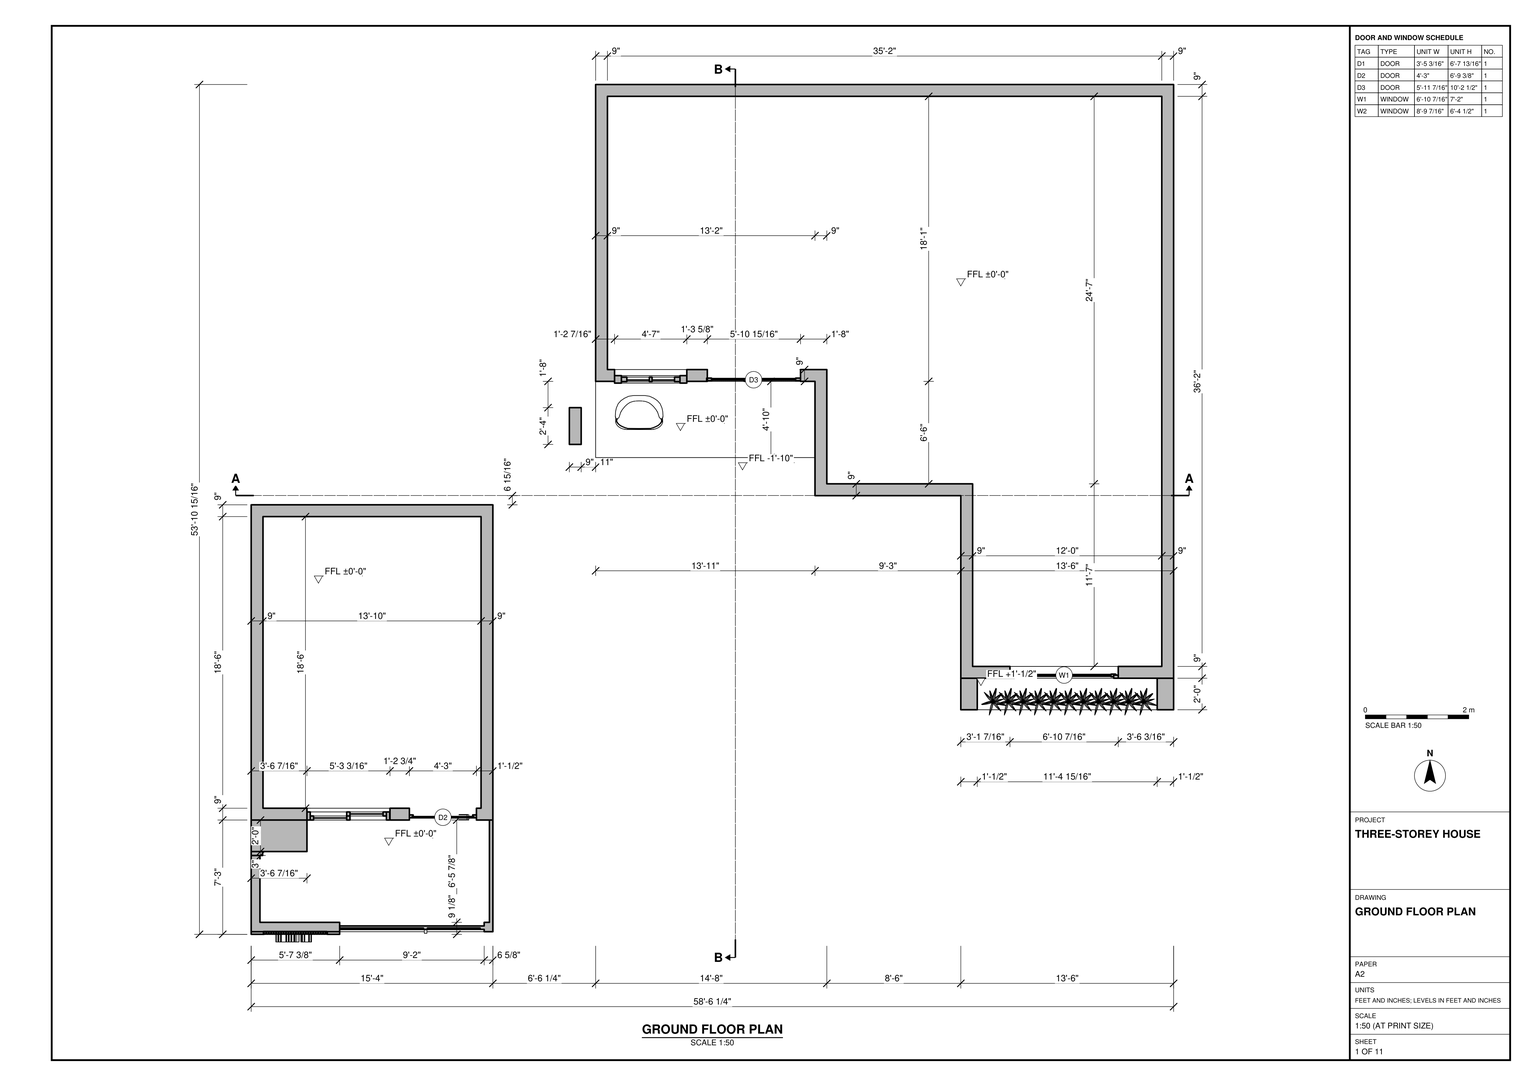
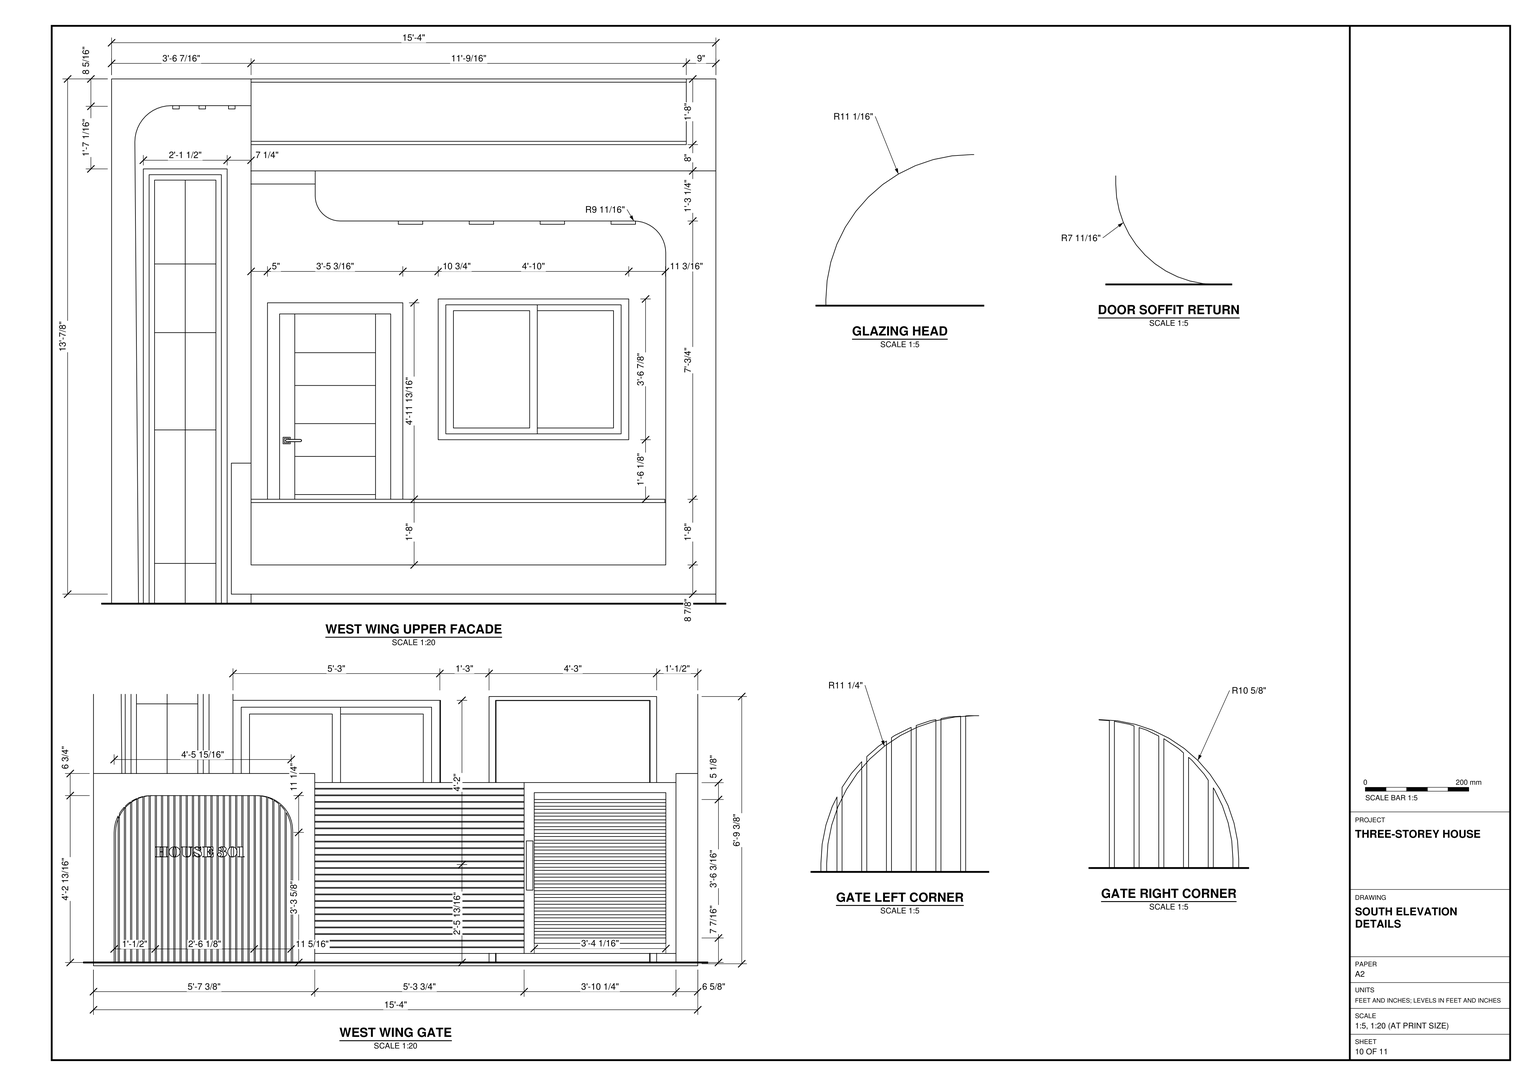
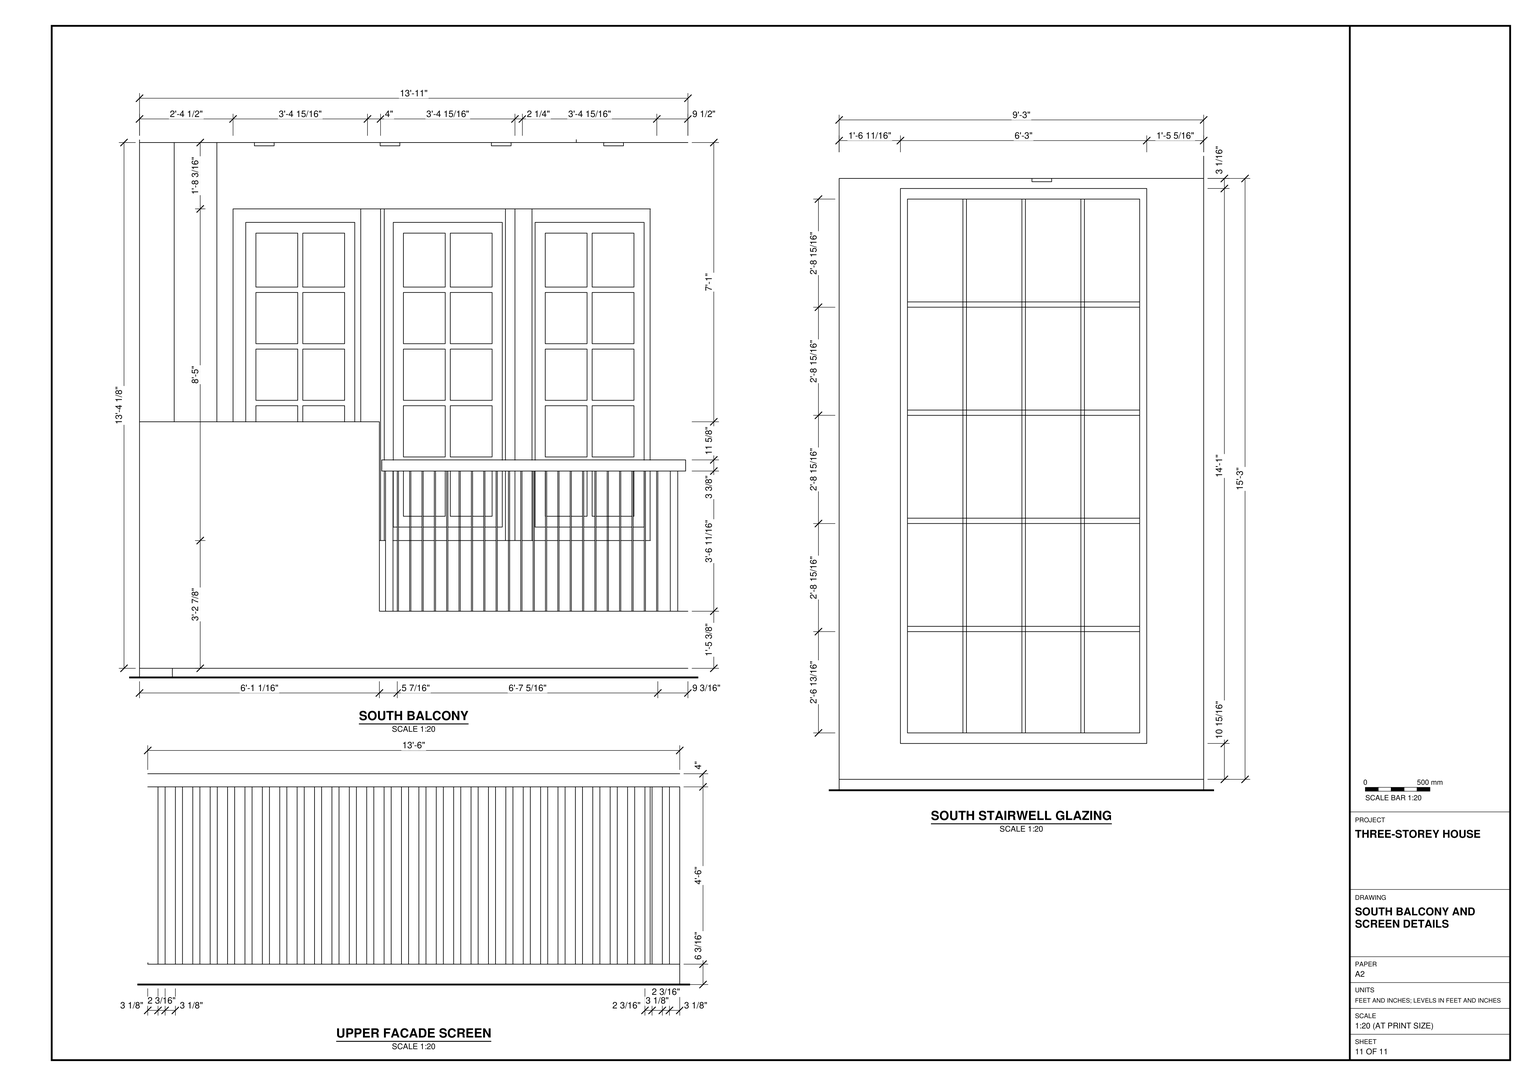
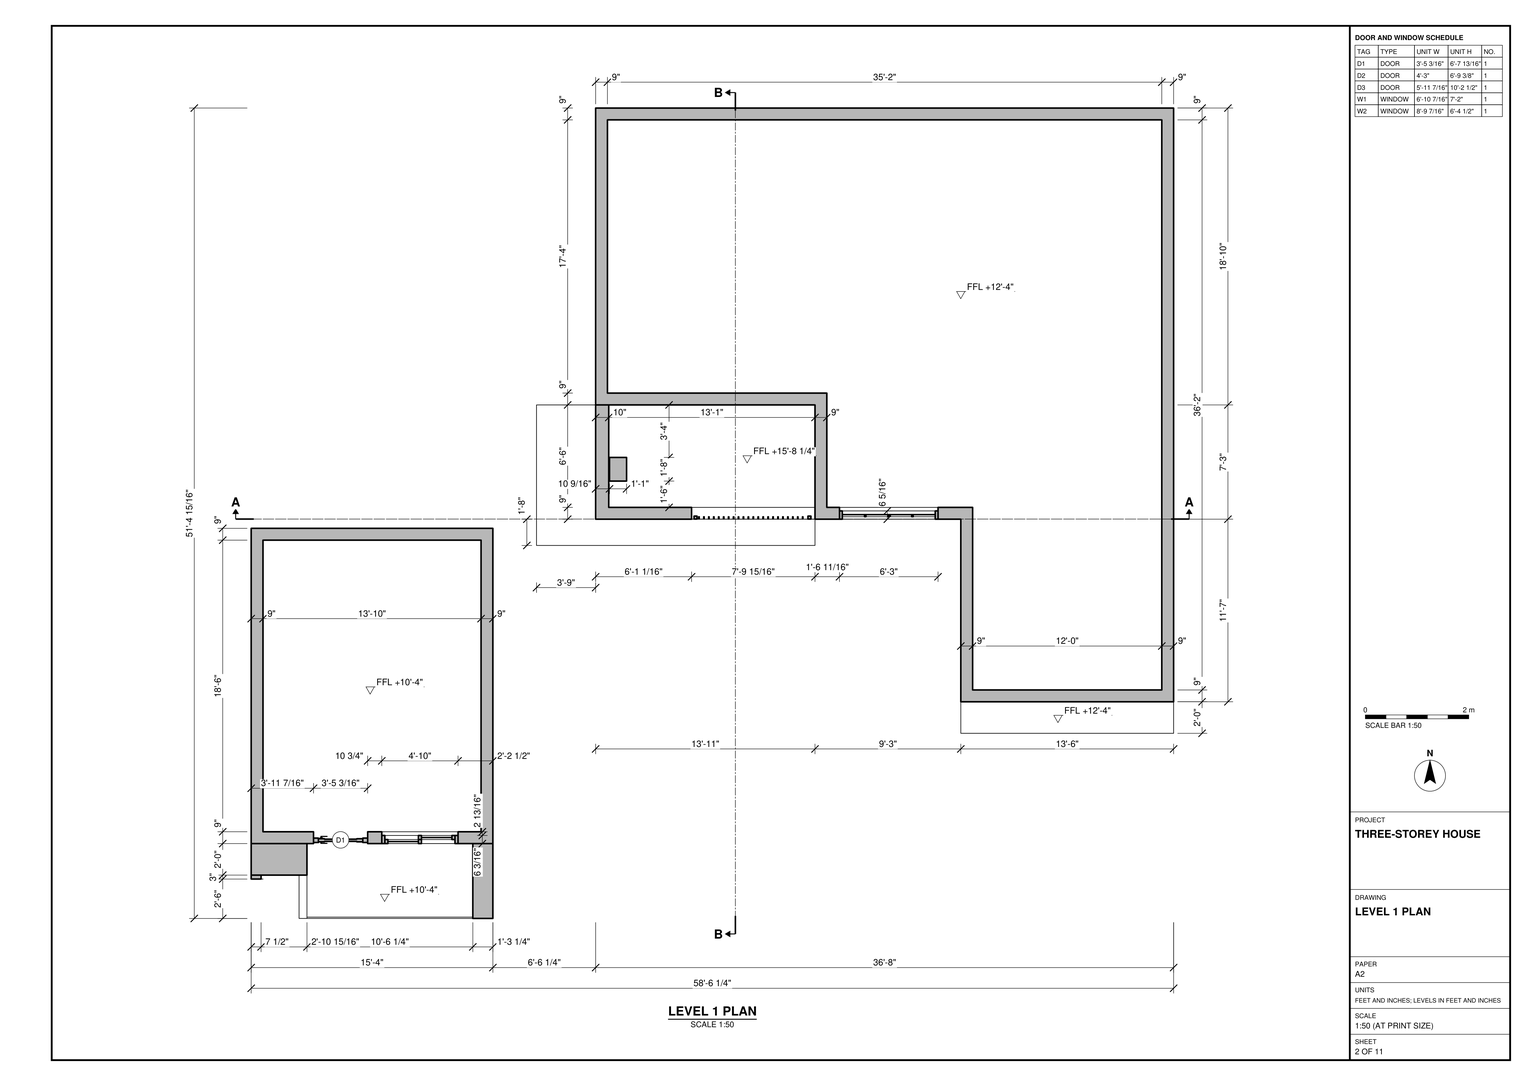
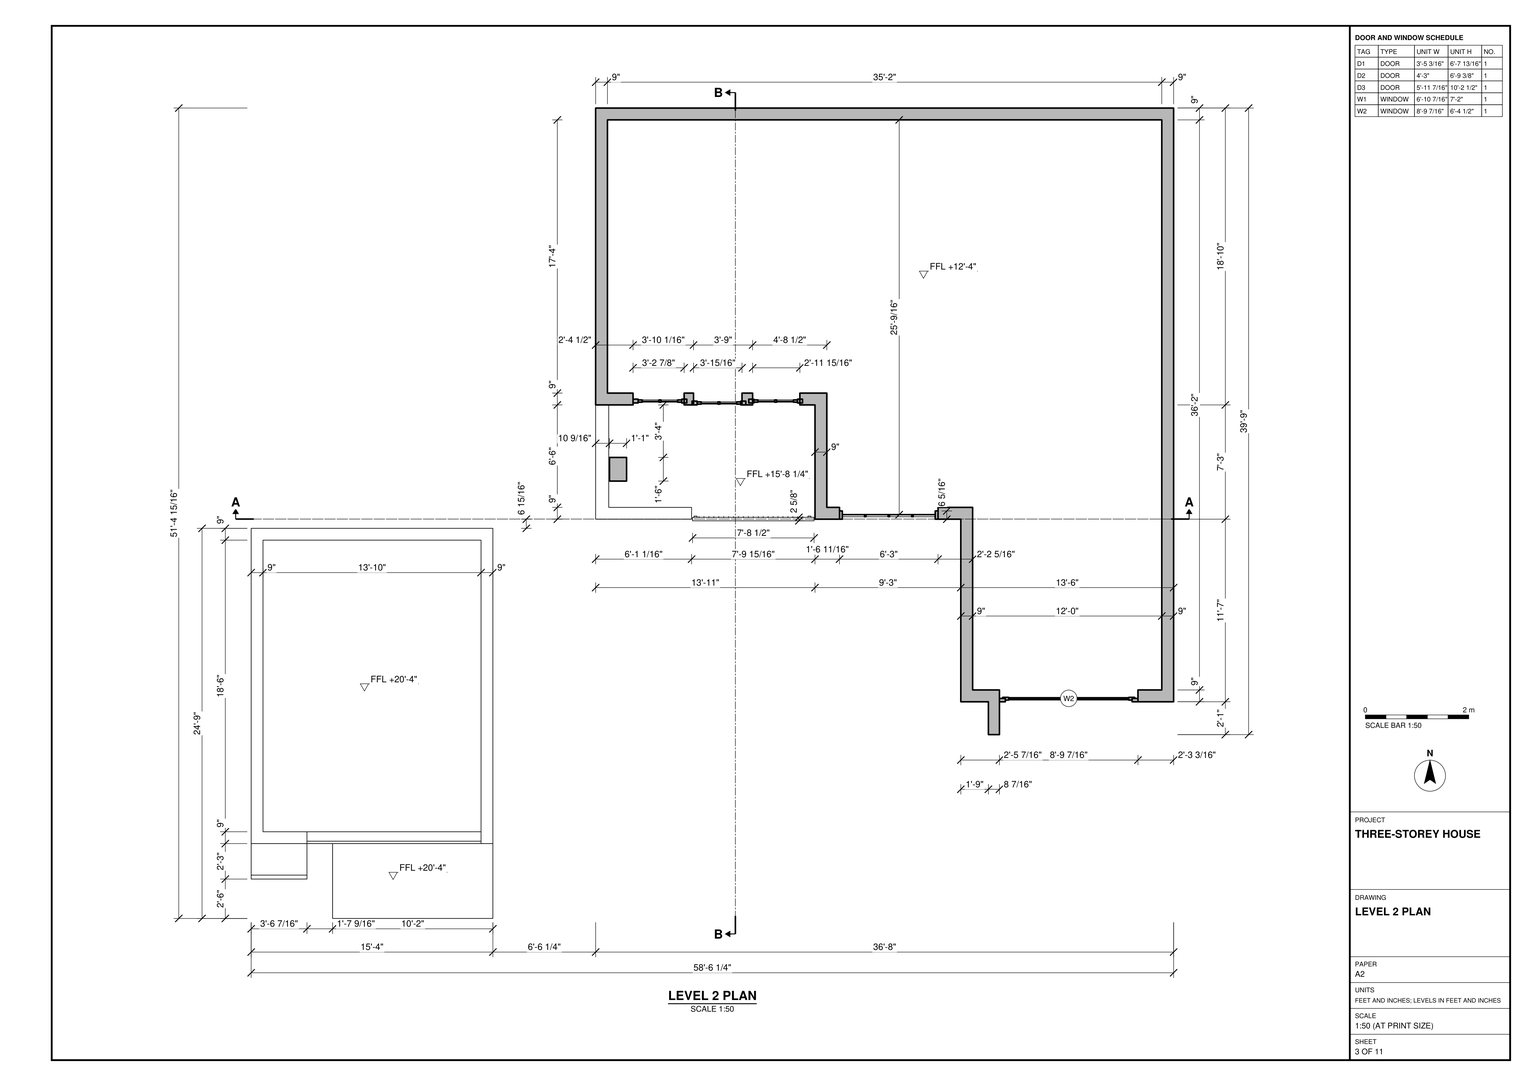
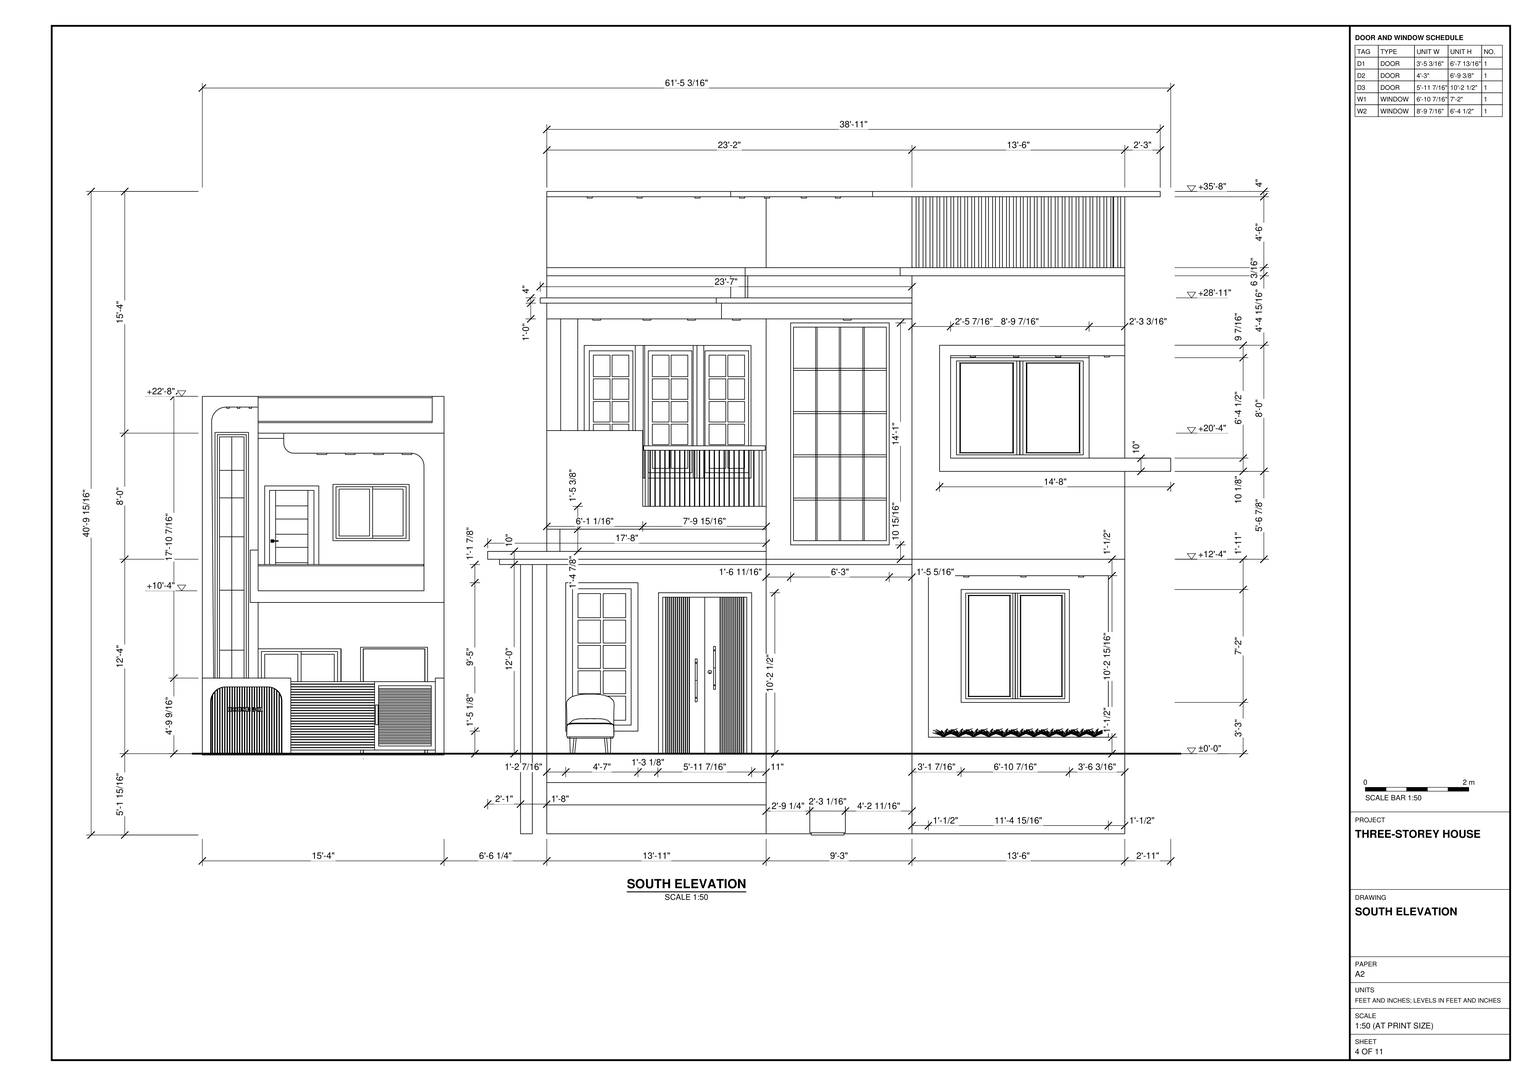
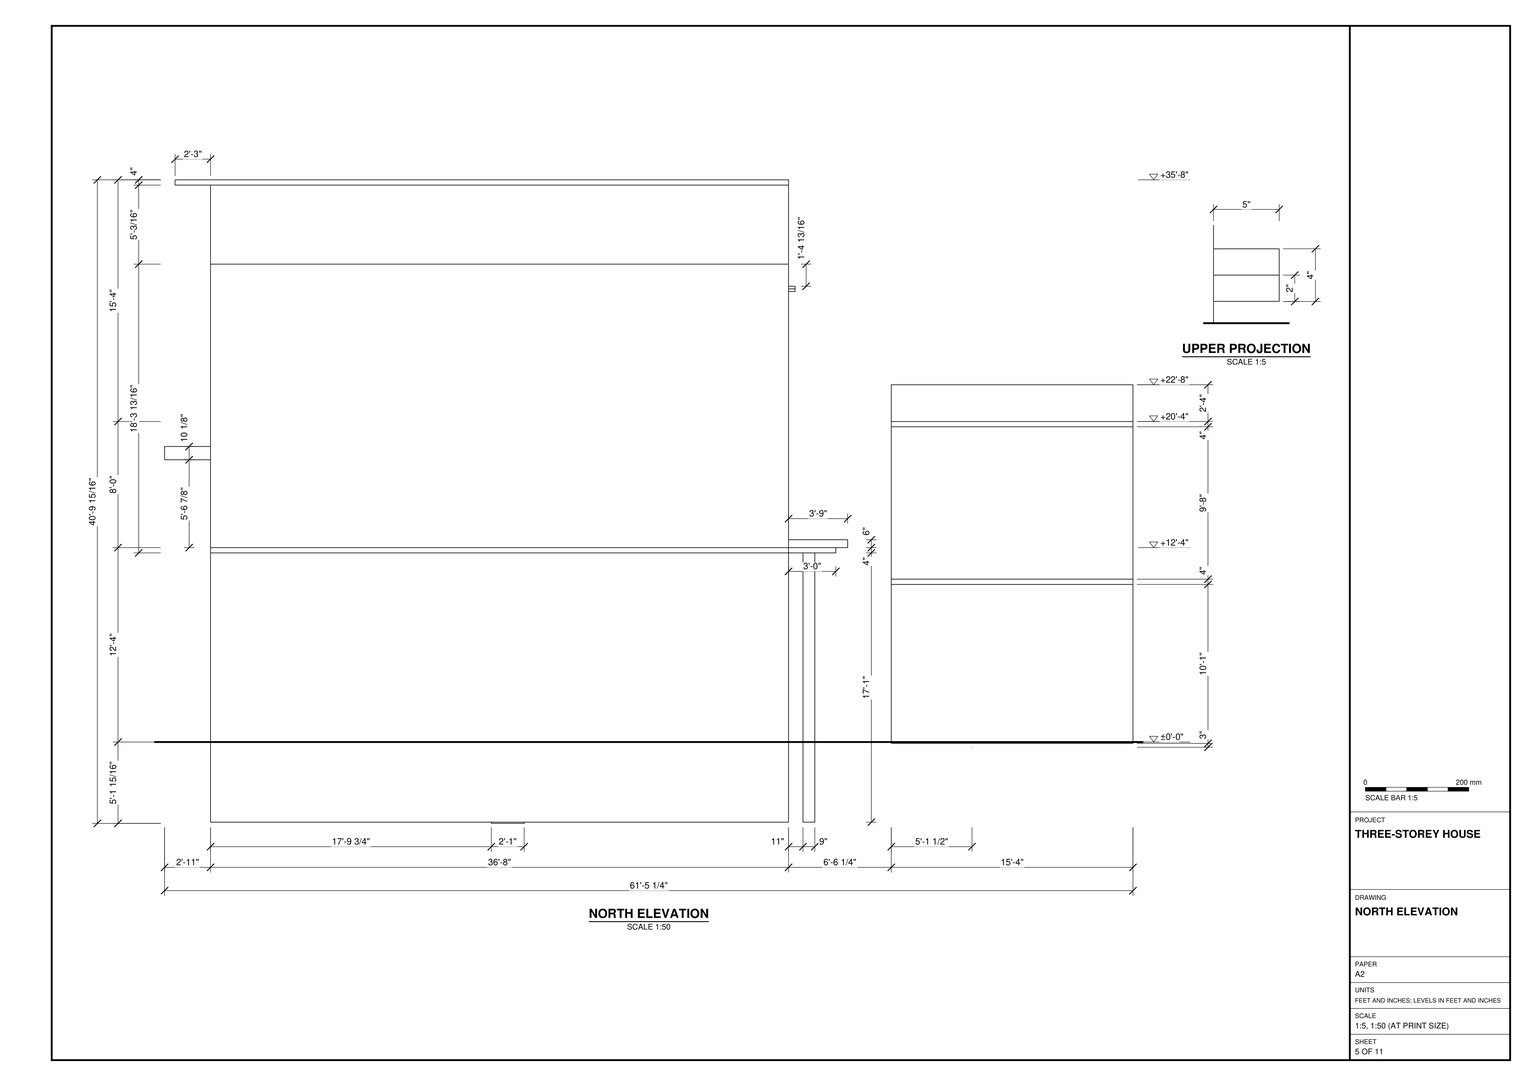
Build the three-storey house in SketchUp from task_files/diagram_01.pdf. Work in feet and inches. The overall model extents are 61'-5 1/4" along X, 56'-7 13/16" along Y and 40'-9 15/16" vertically. Set the storey levels to ±0'-0", +12'-4" and +20'-4" relative to the ground floor.

Lay out the narrow rectangular west wing separately from the larger ground-floor block to its northeast. Follow the stepped outline of the larger block, including the recessed entrance and the projecting bay with planting below its window. Use the wall thicknesses shown in plan, including the 9" perimeter walls. Model the floor slabs, stairs, landings and roof to the plans and sections. Fit the doors and windows into the wall openings using the schedule and elevation details.

Reproduce the slatted west gate and the curved returns around the upper west facade. On the south facade, distinguish the balcony's solid wall from its open railing, and model the divided stairwell glazing and the upper vertical screen. Include the built-in elements and main furniture shown, including the seat at the recessed entrance. Decor and loose items, including plants, may use any suitable library components.

Keep shell elements such as walls, slabs and roof separate as groups or components. Group each furniture or joinery piece separately and use components for repeated parts. Save one SketchUp model as output_files/three_storey_house_with_a_gated_west_wing.skp.

# SketchUp Ruby script. Lengths in inches.
U = 1.inch
M = Sketchup.active_model
def pt(a) = Geom::Point3d.new(a.map { |v| v * U })
def face(e, loops, mat)
  f = e.add_face(loops[0].map { |a| pt(a) })
  loops[1..].each { |l| e.add_face(l.map { |a| pt(a) }).erase! }
  f.material = f.back_material = mat if mat
  f
end
# faces: each face lists its corners as indices into pts; further lists are holes
def faces(e, pts, list, mat = nil) = list.each { |f| face(e, (f[0].is_a?(Array) ? f : [f]).map { |l| l.map { |i| pts[i] } }, mat) }
# xy, xz, yz: faces in a plane at the given z, y or x. An outline is a flat list of corners, or four numbers for a rectangle; further outlines are holes
def ring(l) = l.size == 4 ? [[l[0], l[1]], [l[2], l[1]], [l[2], l[3]], [l[0], l[3]]] : l.each_slice(2).to_a
def flat(e, list, mat, &to3) = list.each { |f| face(e, (f[0].is_a?(Array) ? f : [f]).map { |l| ring(l).map { |u, v| to3.(u, v) } }, mat) }
def xy(e, z, list, mat = nil) = flat(e, list, mat) { |x, y| [x, y, z] }
def xz(e, y, list, mat = nil) = flat(e, list, mat) { |x, z| [x, y, z] }
def yz(e, x, list, mat = nil) = flat(e, list, mat) { |y, z| [x, y, z] }
def lines(e, pts, list) = list.each { |a, b| e.add_line(pt(pts[a]), pt(pts[b])) }
# prism: a flat outline (further loops are holes) pulled along v
def prism(e, loops, v, mat = nil)
  f = face(e, loops, mat); d = Geom::Vector3d.new(v.map { |x| x * U })
  f.pushpull(f.normal.samedirection?(d) ? d.length : -d.length)
end
def box(e, o, s, mat = nil) = prism(e, [[o, [o[0] + s[0], o[1], o[2]], [o[0] + s[0], o[1] + s[1], o[2]], [o[0], o[1] + s[1], o[2]]]], [0, 0, s[2]], mat)
def at(x, y, z, deg = 0) = Geom::Transformation.translation(pt([x, y, z])) * Geom::Transformation.rotation(ORIGIN, Z_AXIS, deg.degrees)
def axes(o, x, y, z) = Geom::Transformation.new([*x, 0, *y, 0, *z, 0, *pt(o).to_a, 1])
def part(name) = M.definitions.add(name)
# library, detail: a bought-in or finely detailed component or shape, given as its bounding box
def library(name, o, s) = part(name).tap { |d| box(d.entities, o, s) }
def detail(e, o, s) = box(e.add_group.entities, o, s)
def put(e, d, t, mat = nil) = e.add_instance(d, t).tap { |i| i.material = mat if mat }
def group(e, t, mat = nil) = e.add_group.tap { |g| g.transformation = t; g.material = mat if mat }.entities
root = M.entities
M.materials.add("Aluminum_Bumpy_5cm\#1").color = [83, 85, 85]
M.materials.add("Heather_Brim").color = [96, 66, 40]
M.materials.add("Heather_Brim1").color = [73, 50, 31]
M.materials.add("Heather_Cuffs").color = [111, 126, 137]
M.materials.add("Heather_Hat").color = [155, 148, 119]
M.materials.add("Lily_Blonde").color = [204, 166, 109]
M.materials.add("Lily_Light").color = [247, 247, 197]
M.materials.add("[Color E05]").color = [255, 255, 0]
M.materials.add("[Color M01]").color = [226, 226, 226]
M.materials.add("[Color M02]").color = [198, 198, 198]
M.materials.add("[Color M09]").color = [0, 0, 0]
M.materials.add("[Formica Speckled Grey]").color = [94, 105, 111]
M.materials.add("[Marble Carrara Floor Tile]").color = [204, 208, 219]
M.materials.add("[Quartz Light Grey]").color = [251, 251, 252]
M.materials.add("[Translucent Glass Blue]").color = [100, 149, 237]
M.materials.add("[Wood Cherry Original]").color = [152, 86, 42]
M.materials.add("[Wood Veneer 01]").color = [120, 70, 37]
c1 = library("Door+01",[0,-2.84,-4],[33.31,7.1,94])
c2 = library("door by lz",[5.91,-4.92,0],[35.43,6.61,78.74])
c3 = library("HOUSE 301",[0.15,0,0],[27.16,3.125,6])
c4 = library("okno",[0,0,0],[1.97,20.83,48.43])
c5 = library("normal+window",[0,0,0],[4.84,65.35,84.65])
c6 = library("modern+double+door",[0,0,0],[3.2,48,90])
c7 = library("BANK+STOEL+MET+RONDE+LEUNING",[-13.09,-13.32,0],[26.18,25.9,25.63])
c8 = library("Plant",[0,0,0],[12.59,12.59,14.16])
c9 = part("Difference\#1")
xy(c9.entities,0,[[0,0,0,240,184,240,184,0,171.48,0,171.48,9,175,9,175,231,9,231,9,9,47.47,9,47.47,0],[47.47,0,88.68,9],[88.68,0,171.48,9]],"Lily_Blonde")
xy(c9.entities,79.83,[[47.47,0,88.68,9]],"Lily_Blonde")
xy(c9.entities,81,[[99.45,0,157.48,9]],"Lily_Blonde")
xy(c9.entities,128,[[42.47,0,175,9]],"[Quartz Light Grey]")
xy(c9.entities,148,[[0,0,42.47,0,42.47,9,9,9,9,231,175,231,175,0,184,0,184,240,0,240]],"[Quartz Light Grey]")
xz(c9.entities,0,[[[42.47,0,47.47,0,47.47,79.83,88.68,79.83,88.68,0,184,0,184,148,175,148,175,128,42.47,128],[99.45,38.13,157.48,81]]],"[Color M01]")
xz(c9.entities,9,[[[9,0,9,148,42.47,148,42.47,128,175,128,175,0,88.68,0,88.68,79.83,47.47,79.83,47.47,0],[99.45,40.5,157.48,81]]],"[Quartz Light Grey]")
xz(c9.entities,231,[[9,0,175,148]],"[Quartz Light Grey]")
xz(c9.entities,240,[[0,0,184,148]],"[Quartz Light Grey]")
yz(c9.entities,0,[[0,0,240,148]],"[Quartz Light Grey]")
yz(c9.entities,9,[[9,0,231,148]],"[Quartz Light Grey]")
yz(c9.entities,42.47,[[0,128,9,148]],"[Quartz Light Grey]")
yz(c9.entities,47.47,[[0,0,9,79.83]],"Lily_Blonde")
yz(c9.entities,88.68,[[0,0,9,79.83]],"Lily_Blonde")
yz(c9.entities,99.45,[[0,38.13,9,40.5,9,81,0,81]],"Lily_Blonde")
yz(c9.entities,157.48,[[0,38.13,0,81,9,81,9,40.5]],"Lily_Blonde")
yz(c9.entities,175,[[9,0,231,148],[0,128,9,148]],"Lily_Blonde")
yz(c9.entities,184,[[0,0,240,148]],"[Quartz Light Grey]")
p = [[99.45,9,40.5],[99.45,0,38.13],[157.48,0,38.13],[157.48,9,40.5]]
faces(c9.entities,p,[[0,1,2,3]],"Lily_Blonde")
c10 = part("Group\#7")
box(c10.entities,[0,0,0],[132.53,1.81,1])
c11 = part("Group\#8")
xy(c11.entities,0,[[0,0,19.69,39.37]])
c12 = part("Group\#9")
prism(c12.entities,[[[45.28,43.31,0],[45.28,0,0],[21.65,0,0],[21.65,43.31,0]],[[23.62,41.34,0],[23.62,1.97,0],[43.31,1.97,0],[43.31,41.34,0]]],[0,0,1.97])
c13 = part("Group\#13")
g1 = group(c13.entities,at(1.97,1.97,0))
put(g1,c11,at(1.97,1.97,0.98),"[Translucent Glass Blue]")
put(g1,c12,at(-21.65,0,0))
g2 = group(c13.entities,at(23.62,1.97,1.97))
put(g2,c11,at(1.97,1.97,0.98),"[Translucent Glass Blue]")
put(g2,c12,at(-21.65,0,0))
g3 = group(c13.entities,at(0,0,3.9375))
prism(g3,[[[0,47.24,-3.9375],[49.21,47.24,-3.9375],[49.21,0,-3.9375],[0,0,-3.9375]],[[1.97,1.97,-3.9375],[47.24,1.97,-3.9375],[47.24,45.28,-3.9375],[1.97,45.28,-3.9375]]],[0,0,3.9375])
c14 = library("Group\#3",[0,-27,0],[42.47,27,272])
c15 = library("Group\#15",[-257.96,-2,-32.54],[67.37,2,57.55])
c16 = library("Group\#16",[13.45,-2,0],[53.92,2,50.83])
c17 = part("Horizontal slat")
xy(c17.entities,0,[[0,0,63.76,1]])
xy(c17.entities,1.75,[[0,0,63.76,1]],"Heather_Brim")
xz(c17.entities,0,[[0,0,63.76,1.75]],"Heather_Brim")
xz(c17.entities,1,[[0,0,63.76,1.75]])
yz(c17.entities,0,[[0,0,1,1.75]])
yz(c17.entities,63.76,[[0,0,1,1.75]])
c18 = part("Group\#20")
put(c18.entities,c17,at(0,-1,0))
c19 = library("Group\#19",[0,-1,-41.22],[40.08,1.95,42.17])
c20 = part("Difference\#2")
xy(c20.entities,0,[[0,-85,0,-27,6.6875,-27,6.6875,-77.875,63.37,-77.875,63.37,-85],[63.37,-85,67.37,-77.875],[177.37,-85,177.37,-77.875,181.37,-77.875,181.37,0,184,0,184,-85],[0,0,0,240,184,240,184,0,171.48,0,171.48,9,175,9,175,231,9,231,9,9,120.45,9,120.45,0]])
xy(c20.entities,2.75,[[131.125,-83.25,131.125,-82.25,67.37,-82.25,67.37,-80.625,177.37,-80.625,177.37,-83.25]])
xy(c20.entities,5.83,[[134.21,-83.25,174.29,-82.25]])
xy(c20.entities,29.83,[[42.47,0,105.68,9]])
xy(c20.entities,51.72,[[134.21,-83.25,174.29,-82.25]])
xy(c20.entities,54.8,[[131.125,-83.25,177.37,-83.25,177.37,-80.625,67.37,-80.625,67.37,-82.25,131.125,-82.25]])
xy(c20.entities,57.55,[[0,-85,63.37,-85,63.37,-77.875,6.6875,-77.875,6.6875,-27,0,-27],[63.37,-85,67.37,-77.875],[177.37,-85,184,-85,184,0,181.37,0,181.37,-77.875,177.37,-77.875]])
xy(c20.entities,79.83,[[42.47,0,105.68,9]])
xy(c20.entities,81,[[120.45,0,171.48,9]])
xy(c20.entities,115.1,[[36.47,-57,36.47,-24,42.47,-24,42.47,0,184,0,184,-57]],"[Formica Speckled Grey]")
xy(c20.entities,124,[[42.47,-57,168.74,0],[168.74,-57,171.48,0],[171.48,-57,184,0]])
xy(c20.entities,155,[[36.47,-57,42.47,-24]],"[Formica Speckled Grey]")
xy(c20.entities,228.74,[[69.63,-57,159.02,0]],"[Formica Speckled Grey]")
xy(c20.entities,244,[[62,-57,184,0]],"[Formica Speckled Grey]")
xz(c20.entities,-85,[[0,0,67.37,57.55],[177.37,0,184,57.55]])
xz(c20.entities,-83.25,[[[131.125,2.75,177.37,54.8],[134.21,5.83,174.29,51.72]]],"Heather_Hat")
xz(c20.entities,-82.25,[[67.37,2.75,131.125,53.05]])
xz(c20.entities,-82.25,[[134.21,5.83,174.29,48.6875],[134.21,49.64,174.29,51.72]],"Heather_Hat")
xz(c20.entities,-80.625,[[67.37,2.75,177.37,54.8]])
xz(c20.entities,-77.875,[[6.6875,0,63.37,57.55],[63.37,0,67.37,57.55],[177.37,0,181.37,57.55]])
xz(c20.entities,-57,[[36.47,115.1,184,115.1,184,124,42.47,124,42.47,155,36.47,155],[168.74,124,184,124,184,244,62,244,62,236.37,62.07,235.37,62.26,234.39,62.58,233.45,63.02,232.55,63.58,231.72,64.24,230.97,64.99,230.3125,65.82,229.76,66.71,229.32,67.66,229,68.64,228.8,69.63,228.74,159.02,228.74,160.29,228.65,161.54,228.41,162.74,228,163.88,227.4375,164.9375,226.73,165.89,225.89,166.73,224.9375,167.4375,223.88,168,222.74,168.41,221.54,168.65,220.29,168.74,219.02]],"[Formica Speckled Grey]")
xz(c20.entities,-27,[[0,0,6.6875,57.55]])
xz(c20.entities,-24,[[36.47,115.1,42.47,155]])
xz(c20.entities,0,[[0,0,42.47,120],[42.47,0,120.45,0,120.45,81,171.48,81,171.48,0,181.37,0,181.37,57.55,184,57.55,184,115.1,42.47,115.1,42.47,79.83,105.68,79.83,105.68,29.83,42.47,29.83],[181.37,0,184,57.55],[168.74,124,168.74,219.02,168.65,220.29,168.41,221.54,168,222.74,167.4375,223.88,166.73,224.9375,165.89,225.89,164.9375,226.73,163.88,227.4375,162.74,228,161.54,228.41,160.29,228.65,159.02,228.74,69.63,228.74,68.64,228.8,67.66,229,66.71,229.32,65.82,229.76,64.99,230.3125,64.24,230.97,63.58,231.72,63.02,232.55,62.58,233.45,62.26,234.39,62.07,235.37,62,236.37,62,244,184,244,184,124]])
xz(c20.entities,9,[[[9,0,9,120,175,120,175,0,171.48,0,171.48,81,120.45,81,120.45,0],[42.47,29.83,105.68,79.83]]])
xz(c20.entities,231,[[9,0,175,120]])
xz(c20.entities,240,[[0,0,184,120]])
yz(c20.entities,0,[[-85,0,-27,57.55],[0,0,240,120]])
yz(c20.entities,6.6875,[[-77.875,0,-27,57.55]])
yz(c20.entities,9,[[9,0,231,120]])
yz(c20.entities,36.47,[[-57,115.1,-24,155]],"[Formica Speckled Grey]")
yz(c20.entities,42.47,[[0,29.83,9,79.83],[-24,115.1,0,124]])
yz(c20.entities,42.47,[[-57,124,-24,155]],"[Formica Speckled Grey]")
yz(c20.entities,62,[[-57,236.37,0,244]],"[Formica Speckled Grey]")
yz(c20.entities,67.37,[[[-85,0,-77.875,57.55],[-82.25,2.75,-80.625,54.8]],[-82.25,2.75,-80.625,54.8]])
yz(c20.entities,105.68,[[0,29.83,9,79.83]])
yz(c20.entities,120.45,[[0,0,9,81]])
yz(c20.entities,131.125,[[-83.25,2.75,-82.25,53.05],[-83.25,53.05,-82.25,54.8]])
yz(c20.entities,134.21,[[-83.25,5.83,-82.25,51.72]])
yz(c20.entities,168.74,[[-57,124,0,219.02]],"[Formica Speckled Grey]")
yz(c20.entities,171.48,[[0,0,9,81]])
yz(c20.entities,174.29,[[-83.25,5.83,-82.25,51.72]])
yz(c20.entities,175,[[9,0,231,120]])
yz(c20.entities,177.37,[[[-85,0,-77.875,57.55],[-83.25,2.75,-80.625,54.8]]])
yz(c20.entities,181.37,[[-77.875,0,0,57.55]])
yz(c20.entities,184,[[-85,0,0,57.55],[0,0,240,0,240,120,-57,120,-57,115.1,0,115.1],[-57,120,0,124]])
yz(c20.entities,184,[[-57,124,0,244]],"[Formica Speckled Grey]")
p = [[168.74,-57,219.02],[168.65,-57,220.29],[168.65,0,220.29],[168.74,0,219.02],[168.41,-57,221.54],[168.41,0,221.54],
  [168,-57,222.74],[168,0,222.74],[167.4375,-57,223.88],[167.4375,0,223.88],[166.73,-57,224.9375],[166.73,0,224.9375],
  [165.89,-57,225.89],[165.89,0,225.89],[164.9375,-57,226.73],[164.9375,0,226.73],[163.88,-57,227.4375],[163.88,0,227.4375],
  [162.74,-57,228],[162.74,0,228],[161.54,-57,228.41],[161.54,0,228.41],[160.29,-57,228.65],[160.29,0,228.65],
  [69.63,-57,228.74],[68.64,-57,228.8],[68.64,0,228.8],[69.63,0,228.74],[159.02,-57,228.74],[159.02,0,228.74],
  [67.66,-57,229],[67.66,0,229],[66.71,-57,229.32],[66.71,0,229.32],[65.82,-57,229.76],[65.82,0,229.76],
  [64.99,-57,230.3125],[64.99,0,230.3125],[64.24,-57,230.97],[64.24,0,230.97],[63.58,-57,231.72],[63.58,0,231.72],
  [63.02,-57,232.55],[63.02,0,232.55],[62.58,-57,233.45],[62.58,0,233.45],[62.26,-57,234.39],[62.26,0,234.39],
  [62.07,-57,235.37],[62.07,0,235.37],[62,-57,236.37],[62,0,236.37]]
faces(c20.entities,p,[[0,1,2,3],[1,4,5,2],[4,6,7,5],[6,8,9,7],[8,10,11,9],[10,12,13,11],[12,14,15,13],[14,16,17,15],
  [16,18,19,17],[18,20,21,19],[20,22,23,21],[24,25,26,27],[22,28,29,23],[25,30,31,26],[30,32,33,31],[32,34,35,33],
  [34,36,37,35],[36,38,39,37],[38,40,41,39],[40,42,43,41],[42,44,45,43],[44,46,47,45],[46,48,49,47],[48,50,51,49]],"[Formica Speckled Grey]")
put(c20.entities,c14,at(0,0,0))
put(c20.entities,c15,at(257.96,-85,32.54),"Aluminum_Bumpy_5cm\#1")
put(c20.entities,c16,at(-7.16,-84.84,0),"Heather_Brim1")
g4 = group(c20.entities,at(67.37,-82.25,53.05))
put(g4,c17,at(0,-1,0))
put(c20.entities,c18,at(67.37,-82.25,51.04))
put(c20.entities,c18,at(67.37,-82.25,49.03))
put(c20.entities,c18,at(67.37,-82.25,47.01))
put(c20.entities,c18,at(67.37,-82.25,45))
put(c20.entities,c18,at(67.37,-82.25,42.99))
put(c20.entities,c18,at(67.37,-82.25,40.98))
put(c20.entities,c18,at(67.37,-82.25,38.97))
put(c20.entities,c18,at(67.37,-82.25,36.95))
put(c20.entities,c18,at(67.37,-82.25,34.94))
put(c20.entities,c18,at(67.37,-82.25,32.93))
put(c20.entities,c18,at(67.37,-82.25,30.92))
put(c20.entities,c18,at(67.37,-82.25,28.91))
put(c20.entities,c18,at(67.37,-82.25,26.89))
put(c20.entities,c18,at(67.37,-82.25,24.88))
put(c20.entities,c18,at(67.37,-82.25,22.87))
put(c20.entities,c18,at(67.37,-82.25,20.86))
put(c20.entities,c18,at(67.37,-82.25,18.85))
put(c20.entities,c18,at(67.37,-82.25,16.83))
put(c20.entities,c18,at(67.37,-82.25,14.82))
put(c20.entities,c18,at(67.37,-82.25,12.81))
put(c20.entities,c18,at(67.37,-82.25,10.8))
put(c20.entities,c18,at(67.37,-82.25,8.79))
put(c20.entities,c18,at(67.37,-82.25,6.77))
put(c20.entities,c18,at(67.37,-82.25,4.76))
put(c20.entities,c18,at(67.37,-82.25,2.75))
put(c20.entities,c19,at(134.21,-82.25,48.6875))
c21 = part("Difference")
xy(c21.entities,0,[[278,0,278,139,167,139,167,226,155.98,226,155.98,235,176,235,176,148,287,148,287,9,431,9,431,443,9,443,9,235,85.04,235,85.04,226,0,226,0,452,440,452,440,0]])
xy(c21.entities,17.15,[[14.41,226,69.41,235]])
xy(c21.entities,39,[[315.41,0,397.84,9]])
xy(c21.entities,122.51,[[85.04,226,155.98,235]])
xy(c21.entities,125,[[315.41,0,397.84,9]])
xy(c21.entities,130.15,[[14.41,226,69.41,235]])
xy(c21.entities,144,[[[278,0,440,0,440,452,0,452,0,226,167,226,167,139,278,139],[287,9,287,148,176,148,176,235,9,235,9,443,431,443,431,9]]])
xz(c21.entities,0,[[[278,0,440,144],[315.41,39,397.84,125]]])
xz(c21.entities,9,[[[287,0,431,144],[315.41,39,397.84,125]]])
xz(c21.entities,139,[[167,0,278,144]])
xz(c21.entities,148,[[176,0,287,144]])
xz(c21.entities,226,[[[0,0,85.04,0,85.04,122.51,155.98,122.51,155.98,0,167,0,167,144,0,144],[14.41,17.15,69.41,130.15]],[0,144,167,148]])
xz(c21.entities,235,[[[9,0,9,144,176,144,176,0,155.98,0,155.98,122.51,85.04,122.51,85.04,0],[14.41,17.15,69.41,130.15]]])
xz(c21.entities,443,[[9,0,431,144]])
xz(c21.entities,452,[[0,0,440,144]])
yz(c21.entities,0,[[226,0,452,144]])
yz(c21.entities,9,[[235,0,443,144]])
yz(c21.entities,14.41,[[226,17.15,235,130.15]])
yz(c21.entities,69.41,[[226,17.15,235,130.15]])
yz(c21.entities,85.04,[[226,0,235,122.51]])
yz(c21.entities,155.98,[[226,0,235,122.51]])
yz(c21.entities,167,[[139,0,226,144]])
yz(c21.entities,176,[[148,0,235,144]])
yz(c21.entities,278,[[0,0,139,144]])
yz(c21.entities,287,[[9,0,148,144]])
yz(c21.entities,315.41,[[0,39,9,125]])
yz(c21.entities,397.84,[[0,39,9,125]])
yz(c21.entities,431,[[9,0,443,144]])
yz(c21.entities,440,[[0,0,452,144]])
c22 = library("Difference\#3",[-5,-25,0],[480,477,276])
c23 = part("Group43\#1")
box(c23.entities,[916.08,245.78,188.26],[2.36,2.36,22.23])
c24 = part("Group44\#1")
box(c24.entities,[1010.04,245.78,188.26],[2.36,2.36,22.23])
c25 = part("Group46\#1")
box(c25.entities,[916.08,245.58,210.49],[96.32,2.75,1.77])
c26 = library("Group47\#1",[920.98,246.17,188.26],[82.61,1.57,22.23])
c27 = library("Group\#30",[0,0,0],[55.12,3.15,82.68])
c28 = library("Group\#55",[0,0,0],[4,4,1])
c29 = library("Group\#54",[0,0,0],[4,4,1])
c30 = library("Group\#56",[0,0,0],[4,4,1])
c31 = library("Group\#53",[0,0,0],[4,4,1])
c32 = library("Group\#52",[0,0,0],[4,4,1])
c33 = library("Group\#51",[0,0,0],[4,4,1])
c34 = library("Group\#50",[0,0,0],[4,4,1])
c35 = library("Group\#49",[0,0,0],[4,4,1])
c36 = library("Group\#48",[0,0,0],[4,4,1])
c37 = library("Group\#75",[0,0,0],[83.03,75.61,78.48])
box(root,[0,2,-1],[184,325,1])
xy(root,-61,[[540.22,194.96,540.22,333.96,429.22,333.96,429.22,420.96,262.22,420.96,262.22,646.96,702.22,646.96,702.22,194.96],[262.22,312.18,429.22,420.96],[242.22,372.96,251.22,400.96]])
xy(root,-39,[[262.22,312.18,429.22,333.18]],"[Marble Carrara Floor Tile]")
xy(root,-22,[[262.22,333.18,429.22,362.96]],"[Marble Carrara Floor Tile]")
xy(root,0,[[540.22,194.96,702.22,194.96,702.22,646.96,262.22,646.96,262.22,420.96,429.22,420.96,429.22,333.96,540.22,333.96]])
xy(root,0,[[262.22,362.96,429.22,420.96]],"[Marble Carrara Floor Tile]")
xy(root,22.04,[[131.8,0.75,133.8,3.75]],"[Color M09]")
xy(root,37.04,[[131.8,0.75,133.8,3.75]],"[Color M09]")
xy(root,143,[[42.47,30,168.47,31]],"[Wood Veneer 01]")
xy(root,144,[[242.22,372.96,251.22,400.96]])
xy(root,144,[[42.47,30,168.47,31]],"[Wood Veneer 01]")
xy(root,148,[[272.22,401.96,429.22,420.96]])
xy(root,170.89,[[262.22,333.96,272.22,420.96],[272.22,333.96,429.22,401.96],[272.22,401.96,429.22,420.96]])
xy(root,188.26,[[335.26,333.96,429.22,342.96],[[272.2,342.96,429.22,420.96],[272.78,362.97,285.78,380.97]]])
xy(root,245.97,[[262.22,333.96,335.26,333.96,335.26,342.96,272.2,342.96,272.2,420.96,262.22,420.96]])
xy(root,331,[[272.78,362.97,285.78,380.97]])
xy(root,424,[[[510.22,151.96,510.22,306.96,402.22,306.96,402.22,393.96,262.22,393.96,262.22,673.96,729.22,673.96,729.22,151.96],[523.35,165.08,716.09,165.08,716.09,660.83,275.35,660.83,275.35,407.08,415.35,407.08,415.35,320.08,523.35,320.08]],[526.88,168.61,526.88,323.61,418.88,323.61,418.88,410.61,278.88,410.61,278.88,657.3,712.5625,657.3,712.5625,168.61]],"[Wood Cherry Original]")
xy(root,427,[[[523.35,165.08,523.35,320.08,415.35,320.08,415.35,407.08,275.35,407.08,275.35,660.83,716.09,660.83,716.09,165.08],[526.88,168.61,712.5625,168.61,712.5625,657.3,278.88,657.3,278.88,410.61,418.88,410.61,418.88,323.61,526.88,323.61]]],"[Color E05]")
xy(root,428,[[510.22,151.96,729.22,151.96,729.22,673.96,262.22,673.96,262.22,393.96,402.22,393.96,402.22,306.96,510.22,306.96]])
xz(root,0.75,[[131.8,22.04,133.8,37.04]],"[Color M09]")
xz(root,3.75,[[131.8,22.04,133.8,37.04]])
xz(root,30,[[42.47,124,168.74,143]],"[Translucent Glass Blue]")
xz(root,30,[[42.47,143,168.47,144]],"[Wood Veneer 01]")
xz(root,31,[[42.47,143,168.47,144]],"[Wood Veneer 01]")
xz(root,87,[[42.47,253,175,271]],"[Translucent Glass Blue]")
xz(root,151.96,[[510.22,424,729.22,428]])
xz(root,165.08,[[523.35,424,716.09,427]])
xz(root,168.61,[[526.88,424,712.5625,427]])
xz(root,194.96,[[540.22,-61,702.22,0]])
xz(root,306.96,[[402.22,424,510.22,428]])
xz(root,312.18,[[262.22,-61,429.22,-39]],"[Marble Carrara Floor Tile]")
xz(root,320.08,[[415.35,424,523.35,427]])
xz(root,323.61,[[418.88,424,526.88,427]])
xz(root,333.18,[[262.22,-39,429.22,-22]],"[Marble Carrara Floor Tile]")
xz(root,333.96,[[429.22,-61,540.22,0],[262.22,170.89,429.22,170.89,429.22,188.26,335.26,188.26,335.26,245.97,262.22,245.97]])
xz(root,342.96,[[272.2,188.26,335.26,245.97]])
xz(root,362.96,[[262.22,-22,429.22,0]],"[Marble Carrara Floor Tile]")
xz(root,362.97,[[272.78,188.26,285.78,331]])
xz(root,372.96,[[242.22,-61,251.22,144]],"Heather_Cuffs")
xz(root,380.97,[[272.78,188.26,285.78,331]])
xz(root,393.96,[[262.22,424,402.22,428]])
xz(root,400.96,[[242.22,-61,251.22,144]])
xz(root,401.96,[[272.22,148,429.22,170.89]])
xz(root,407.08,[[275.35,424,415.35,427]])
xz(root,410.61,[[278.88,424,418.88,427]])
xz(root,420.96,[[262.22,-61,429.22,0],[272.22,148,429.22,170.89],[262.22,188.26,272.2,245.97]])
xz(root,646.96,[[262.22,-61,702.22,0]])
xz(root,657.3,[[278.88,424,712.5625,427]])
xz(root,660.83,[[275.35,424,716.09,427]])
xz(root,673.96,[[262.22,424,729.22,428]])
yz(root,42.47,[[30,143,31,144]],"[Wood Veneer 01]")
yz(root,131.8,[[0.75,22.04,3.75,37.04]],"[Color M09]")
yz(root,133.8,[[0.75,22.04,3.75,37.04]],"[Color M09]")
yz(root,168.47,[[30,143,31,144]],"[Wood Veneer 01]")
yz(root,242.22,[[372.96,-61,400.96,144]])
yz(root,251.22,[[372.96,-61,400.96,144]])
yz(root,262.22,[[312.18,-61,312.18,-39,333.18,-39,333.18,-22,362.96,-22,362.96,0,420.96,0,420.96,-61],[420.96,-61,646.96,0],[333.96,170.89,420.96,245.97],[393.96,424,673.96,428]])
yz(root,272.2,[[342.96,188.26,420.96,245.97]])
yz(root,272.22,[[401.96,148,420.96,170.89]])
yz(root,272.78,[[362.97,188.26,380.97,331]])
yz(root,275.35,[[407.08,424,660.83,427]])
yz(root,278.88,[[410.61,424,657.3,427]])
yz(root,285.78,[[362.97,188.26,380.97,331]])
yz(root,335.26,[[333.96,188.26,342.96,245.97]])
yz(root,402.22,[[306.96,424,393.96,428]])
yz(root,415.35,[[320.08,424,407.08,427]])
yz(root,418.88,[[323.61,424,410.61,427]])
yz(root,429.22,[[312.18,-61,333.96,-61,333.96,-22,333.18,-22,333.18,-39,312.18,-39],[333.96,-61,420.96,-61,420.96,0,362.96,0,362.96,-22,333.96,-22],[333.96,-22,362.96,0],[401.96,148,420.96,170.89],[333.96,170.89,420.96,188.26]])
yz(root,510.22,[[151.96,424,306.96,428]])
yz(root,523.35,[[165.08,424,320.08,427]])
yz(root,526.88,[[168.61,424,323.61,427]])
yz(root,540.22,[[194.96,-61,333.96,0]])
yz(root,702.22,[[194.96,-61,646.96,0]])
yz(root,712.5625,[[168.61,424,657.3,427]])
yz(root,716.09,[[165.08,424,660.83,427]])
yz(root,729.22,[[151.96,424,673.96,428]])
detail(root,[18.61,60.61,262.86],[1.99,1.99,1])
detail(root,[35.61,60.61,262.86],[1.99,1.99,1])
detail(root,[26.61,60.61,262.86],[1.99,1.99,1])
detail(root,[87.3,50.41,227.74],[7.44,7.43,1])
detail(root,[108.9,50.41,227.74],[7.43,7.43,1])
detail(root,[130.49,50.41,227.74],[7.44,7.43,1])
detail(root,[152.09,50.41,227.74],[7.43,7.43,1])
detail(root,[584.58,178.82,302],[4,4,1])
detail(root,[617.58,178.82,302],[4,4,1])
detail(root,[649.58,178.82,302],[4,4,1])
detail(root,[686.58,178.82,302],[4,4,1])
detail(root,[579.55,179.5625,134.48],[4,4,1])
detail(root,[623.07,179.5625,134.48],[4,4,1])
detail(root,[667.07,179.5625,134.48],[4,4,1])
put(root,c1,axes([120.45,88.7,-0.38],[1.53213,0,0],[0,0.59962,0],[0,0,0.90426]))
put(root,c2,axes([40.59,91.1875,124],[1.16305,0,0],[0,0.85119,0],[0,0,1.01386]))
put(root,c3,axes([18.63,0.16,32.12],[1,0,0],[0,0,1],[0,-1,0]),"Lily_Light")
put(root,c4,axes([331.63,419.64,17.15],[0,2.899,0],[-2.64006,0,0],[0,0,2.3335]))
put(root,c4,axes([331.63,422.45,209.8],[0,1.4718,0],[-1.96475,0,0],[0,0,2.08569]))
put(root,c4,axes([376.55,420.96,209.8],[0,1.4718,0],[-1.96475,0,0],[0,0,2.08569]))
put(root,c4,axes([419.74,422.45,209.8],[0,1.4718,0],[-1.96475,0,0],[0,0,2.08569]))
put(root,c5,axes([660.0625,194.96,39],[0,1,0],[-1.26126,0,0],[0,0,1.016]))
put(root,c5,axes([675.0625,194.96,225],[0,1.07568,0],[-1.61319,0,0],[0,0,0.90343]))
put(root,c6,axes([346.76,423.46,0],[0,-0.78125,0],[1.48834,0,0],[0,0,1.36121]))
put(root,c7,axes([295.35,396.87,-0.04],[1.38816,0,0],[0,-1,0],[0,0,1.77]))
put(root,c8,axes([462.45,309.24,-61.95],[2.1504,0,0],[0,2,0],[0,0,2]))
g5 = group(root,at(0,87,120))
g6 = group(g5,at(0,0,-4.9))
xy(g6,4.9,[[0,0,184,240]])
xy(g6,8.9,[[0,0,184,240]])
xz(g6,0,[[42.47,0,184,4.9],[0,4.9,42.47,8.9],[42.47,4.9,184,8.9]])
xz(g6,240,[[0,4.9,184,8.9]])
yz(g6,0,[[0,4.9,240,8.9]])
yz(g6,184,[[0,4.9,240,8.9]])
g7 = group(g5,at(0,0,115.1))
box(g7,[0,0,4.9],[184,240,4])
put(root,c9,at(0,87,124),"[Color M02]")
g8 = group(root,at(42.47,87,252))
put(g8,c10,at(0,0,0),"[Wood Veneer 01]")
put(g8,c10,at(0,0,19),"[Wood Veneer 01]")
put(root,c13,axes([42.47,87,79.83],[1.28,0,0],[0,0,-1.05833],[0,1.56718,0]))
put(root,c13,axes([99.45,87,205],[1.17915,0,0],[0,0,-0.90737],[0,1.56718,0]))
put(root,c20,at(0,87,0))
put(root,c21,at(262.22,194.96,0))
g9 = group(root,at(262.22,194.96,144),"Heather_Cuffs")
xy(g9,0,[[278,0,278,139,167,139,167,130,-36,130,-36,226,0,226,0,452,440,452,440,0]])
xy(g9,4,[[278,0,440,0,440,452,0,452,0,226,1.96,226,1.96,140.7,167,140.7,167,139,278,139],[-45,119,-20,130],[-20,119,-3,130],[-3,119,1.96,130],[1.96,119,167,130],
  [-45,130,-36,226],[-36,130,1.96,226],[1.96,130,167,140.7]])
xy(g9,10,[[-45,119,167,119,167,140.7,1.96,140.7,1.96,226,-45,226]])
xz(g9,0,[[278,0,440,4]])
xz(g9,119,[[-45,4,167,10]])
xz(g9,130,[[-36,0,167,4]])
xz(g9,139,[[167,0,278,4]])
xz(g9,140.7,[[1.96,4,167,10]])
xz(g9,226,[[-36,0,0,4],[-45,4,1.96,10]])
xz(g9,452,[[0,0,440,4]])
yz(g9,-45,[[119,4,226,10]])
yz(g9,-36,[[130,0,226,4]])
yz(g9,0,[[226,0,452,4]])
yz(g9,1.96,[[140.7,4,226,10]])
yz(g9,167,[[130,0,139,4],[119,4,140.7,10]])
yz(g9,278,[[0,0,139,4]])
yz(g9,440,[[0,0,452,4]])
put(root,c22,at(262.22,194.96,148),"Heather_Cuffs")
g10 = group(root,at(540.22,194.96,0))
prism(g10,[[[162,0,0],[0,0,0],[0,0,148],[162,0,148]],[[12.52,0,135.48],[12.52,0,12.52],[149.48,0,12.52],[149.48,0,135.48]]],[0,-24,0],"Heather_Cuffs")
put(root,c23,axes([-542.66,98.01,-173.35],[0.9604,0,0],[0,0.9604,0],[0,0,1.9208]))
put(root,c24,axes([-546.2,98.01,-173.35],[0.9604,0,0],[0,0.9604,0],[0,0,1.9208]))
put(root,c25,axes([-543.8,96.875,-173.35],[0.9604,0,0],[0,0.9604,0],[0,0,1.9208]))
put(root,c26,axes([-543.8,97.83,-173.35],[0.9604,0,0],[0,0.9604,0],[0,0,1.9208]))
put(root,c27,axes([447.88,333.96,158.93],[1.36071,0,0],[0,2,0],[0,0,2.0441]))
put(root,c28,axes([296.91,399.6,424],[-1,0,0],[0,1,0],[0,0,-1]))
put(root,c29,axes([334.91,399.6,424],[-1,0,0],[0,1,0],[0,0,-1]))
put(root,c30,axes([378.91,399.6,424],[-1,0,0],[0,1,0],[0,0,-1]))
put(root,c31,axes([412.91,399.6,424],[-1,0,0],[0,1,0],[0,0,-1]))
put(root,c32,axes([412.91,355.6,424],[-1,0,0],[0,1,0],[0,0,-1]))
put(root,c33,axes([412.91,319.6,424],[-1,0,0],[0,1,0],[0,0,-1]))
put(root,c34,axes([431.86,310.54,424],[-1,0,0],[0,1,0],[0,0,-1]))
put(root,c35,axes([459.86,310.54,424],[-1,0,0],[0,1,0],[0,0,-1]))
put(root,c36,axes([485.86,310.54,424],[-1,0,0],[0,1,0],[0,0,-1]))
put(root,c37,axes([577.56,184.53,12.52],[-0.0659,-0.24592,0],[-0.24592,0.0659,0],[0,0,0.08614]))
put(root,c37,axes([589.03,184.53,12.52],[-0.0659,-0.24592,0],[-0.24592,0.0659,0],[0,0,0.08614]))
put(root,c37,axes([600.5,184.53,12.52],[-0.0659,-0.24592,0],[-0.24592,0.0659,0],[0,0,0.08614]))
put(root,c37,axes([611.97,184.53,12.52],[-0.0659,-0.24592,0],[-0.24592,0.0659,0],[0,0,0.08614]))
put(root,c37,axes([623.44,184.53,12.52],[-0.0659,-0.24592,0],[-0.24592,0.0659,0],[0,0,0.08614]))
put(root,c37,axes([634.91,184.53,12.52],[-0.0659,-0.24592,0],[-0.24592,0.0659,0],[0,0,0.08614]))
put(root,c37,axes([646.38,184.53,12.52],[-0.0659,-0.24592,0],[-0.24592,0.0659,0],[0,0,0.08614]))
put(root,c37,axes([657.86,184.53,12.52],[-0.0659,-0.24592,0],[-0.24592,0.0659,0],[0,0,0.08614]))
put(root,c37,axes([669.33,184.53,12.52],[-0.0659,-0.24592,0],[-0.24592,0.0659,0],[0,0,0.08614]))
put(root,c37,axes([680.8,184.53,12.52],[-0.0659,-0.24592,0],[-0.24592,0.0659,0],[0,0,0.08614]))
put(root,c37,axes([692.27,184.53,12.52],[-0.0659,-0.24592,0],[-0.24592,0.0659,0],[0,0,0.08614]))
